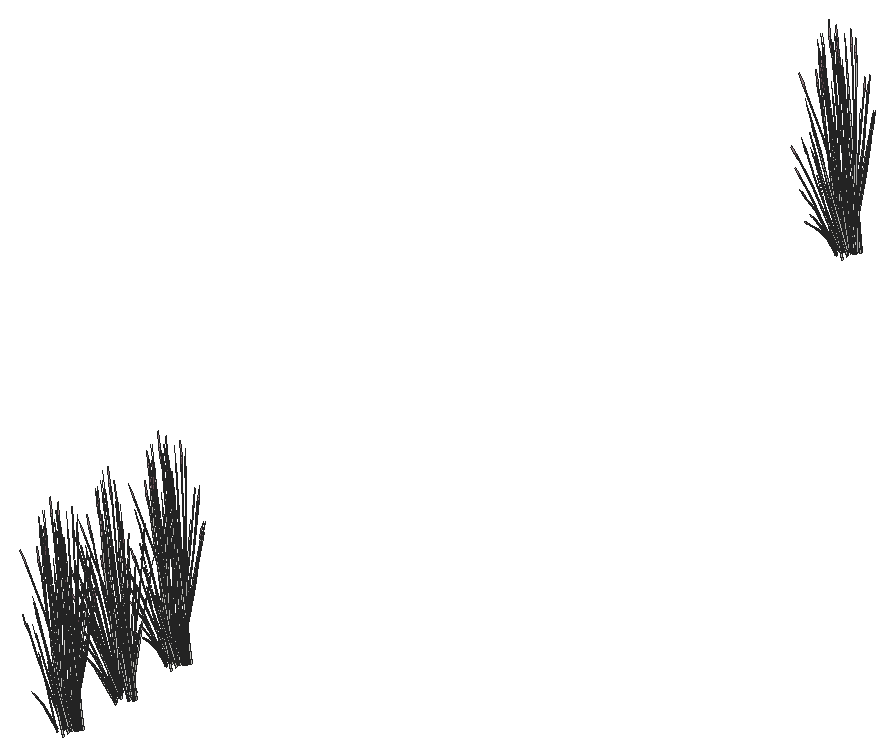
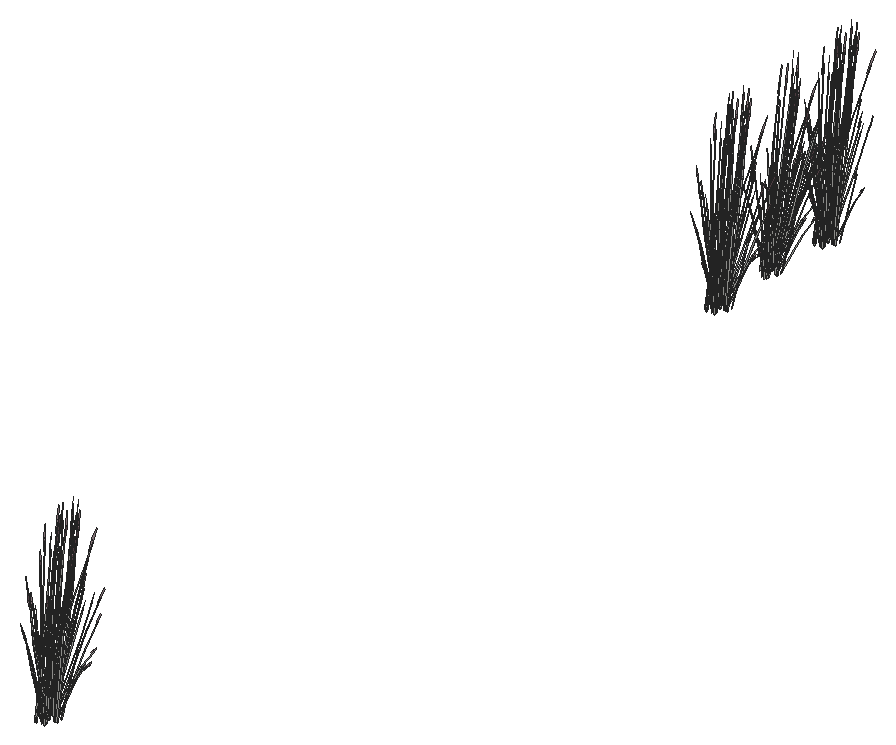
# SketchUp Ruby script. Lengths in inches.
U = 1.inch
M = Sketchup.active_model
def pt(a) = Geom::Point3d.new(a.map { |v| v * U })
def face(e, loops, mat)
  f = e.add_face(loops[0].map { |a| pt(a) })
  loops[1..].each { |l| e.add_face(l.map { |a| pt(a) }).erase! }
  f.material = f.back_material = mat if mat
  f
end
# faces: each face lists its corners as indices into pts; further lists are holes
def faces(e, pts, list, mat = nil) = list.each { |f| face(e, (f[0].is_a?(Array) ? f : [f]).map { |l| l.map { |i| pts[i] } }, mat) }
# xy, xz, yz: faces in a plane at the given z, y or x. An outline is a flat list of corners, or four numbers for a rectangle; further outlines are holes
def ring(l) = l.size == 4 ? [[l[0], l[1]], [l[2], l[1]], [l[2], l[3]], [l[0], l[3]]] : l.each_slice(2).to_a
def flat(e, list, mat, &to3) = list.each { |f| face(e, (f[0].is_a?(Array) ? f : [f]).map { |l| ring(l).map { |u, v| to3.(u, v) } }, mat) }
def xy(e, z, list, mat = nil) = flat(e, list, mat) { |x, y| [x, y, z] }
def xz(e, y, list, mat = nil) = flat(e, list, mat) { |x, z| [x, y, z] }
def yz(e, x, list, mat = nil) = flat(e, list, mat) { |y, z| [x, y, z] }
def lines(e, pts, list) = list.each { |a, b| e.add_line(pt(pts[a]), pt(pts[b])) }
# prism: a flat outline (further loops are holes) pulled along v
def prism(e, loops, v, mat = nil)
  f = face(e, loops, mat); d = Geom::Vector3d.new(v.map { |x| x * U })
  f.pushpull(f.normal.samedirection?(d) ? d.length : -d.length)
end
def box(e, o, s, mat = nil) = prism(e, [[o, [o[0] + s[0], o[1], o[2]], [o[0] + s[0], o[1] + s[1], o[2]], [o[0], o[1] + s[1], o[2]]]], [0, 0, s[2]], mat)
def at(x, y, z, deg = 0) = Geom::Transformation.translation(pt([x, y, z])) * Geom::Transformation.rotation(ORIGIN, Z_AXIS, deg.degrees)
def axes(o, x, y, z) = Geom::Transformation.new([*x, 0, *y, 0, *z, 0, *pt(o).to_a, 1])
def part(name) = M.definitions.add(name)
# library, detail: a bought-in or finely detailed component or shape, given as its bounding box
def library(name, o, s) = part(name).tap { |d| box(d.entities, o, s) }
def detail(e, o, s) = box(e.add_group.entities, o, s)
def put(e, d, t, mat = nil) = e.add_instance(d, t).tap { |i| i.material = mat if mat }
def group(e, t, mat = nil) = e.add_group.tap { |g| g.transformation = t; g.material = mat if mat }.entities
root = M.entities
M.materials.add("LightPink_Translucent").color = [144, 107, 117]
M.materials["LightPink_Translucent"].alpha = 0.75
c1 = part("blade")
p = [[2.15,0.21,22],[0,0.17,0],[0.09,0.45,0],[2.18,0.31,22],[2.29,0.31,22],[0.38,0.45,0],
  [2.48,0.24,33],[2.49,0.24,33],[2.48,0.22,33]]
faces(c1.entities,p,[[0,1,2,3],[4,5,2,3],[6,3,4,7],[8,0,3,6]])
c2 = part("seeds")
p = [[0.3,-0.1,1.38],[-0.01,-0.03,1.59],[-0.01,-0.03,0.03],[0.14,-0.07,-0.07],[0.29,-0.03,3],[0.15,0.01,3.11]]
faces(c2.entities,p,[[0,1,2,3],[1,0,4,5]],"LightPink_Translucent")
c3 = part("blade with seeds")
put(c3.entities,c1,at(0,0,0))
put(c3.entities,c2,axes([2.4,0.25,30.99],[1.5799,-0.05474,1.17369],[-0.12525,1.92788,0.29478],[-0.07173,-0.02425,1.56792]))
put(root,c3,axes([491.625,164.9375,4.29],[0.62747,-0.45094,0.53763],[0.54116,0.47889,0.4433],[-0.29439,-0.08318,1.11249]))
put(root,c3,axes([491.1,167.63,3.92],[-0.52161,-0.25698,0.0643],[0.30368,-0.36595,0.50621],[-0.16723,0.11831,0.77189]))
put(root,c3,axes([488.5,445.23,4.84],[0.67048,0.16311,-0.06488],[-0.20625,0.50201,-0.29416],[-0.10966,0.07622,0.97024]))
put(root,c3,axes([488.57,148.83,4.84],[0.67048,0.16311,-0.06488],[-0.20625,0.50201,-0.29416],[-0.10966,0.07622,0.97024]))
put(root,c3,axes([490,443.81,4.24],[0.66138,-0.08733,0.35414],[0.17464,0.49921,-0.4572],[-0.18953,0.13408,0.87481]))
put(root,c3,axes([488.64,189.9,4.84],[0.67048,0.16311,-0.06488],[-0.20625,0.50201,-0.29416],[-0.10966,0.07622,0.97024]))
put(root,c3,axes([490.08,147.41,4.24],[0.66138,-0.08733,0.35414],[0.17464,0.49921,-0.4572],[-0.18953,0.13408,0.87481]))
put(root,c3,axes([492.16,167.82,3.07],[0.14147,-0.21002,1.71376],[0.59349,0.43464,0.13857],[-0.26773,0.27089,0.73262]))
put(root,c3,axes([490.375,446.1875,1.78],[0.23977,-0.09639,1.43002],[0.59198,0.29065,-0.30754],[-0.1762,0.25149,0.61141]))
put(root,c3,axes([490.14,188.48,4.24],[0.66138,-0.08733,0.35414],[0.17464,0.49921,-0.4572],[-0.18953,0.13408,0.87481]))
put(root,c3,axes([490.04,440.69,1.32],[-0.21918,0.49894,-0.03893],[-0.6746,-0.15348,-0.17649],[-0.10242,-0.08161,0.58215]))
put(root,c3,axes([490.45,149.79,1.78],[0.23977,-0.09639,1.43002],[0.59198,0.29065,-0.30754],[-0.1762,0.25149,0.61141]))
put(root,c3,axes([490.52,190.86,1.78],[0.23977,-0.09639,1.43002],[0.59198,0.29065,-0.30754],[-0.1762,0.25149,0.61141]))
put(root,c3,axes([490.11,144.29,1.32],[-0.21918,0.49894,-0.03893],[-0.6746,-0.15348,-0.17649],[-0.10242,-0.08161,0.58215]))
put(root,c3,axes([491.59,166.36,4.24],[0.63144,0.17046,0.35414],[-0.18417,0.49731,-0.4572],[-0.25423,0.0456,0.87481]))
put(root,c3,axes([490.18,185.36,1.32],[-0.21918,0.49894,-0.03893],[-0.6746,-0.15348,-0.17649],[-0.10242,-0.08161,0.58215]))
put(root,c3,axes([491.79,439,3.9],[-0.01417,0.07324,1.77383],[-0.6991,0.2658,-0.16761],[-0.20573,-0.13587,0.31391]))
put(root,c3,axes([491.04,440.0625,1.78],[-0.04601,0.19989,1.43002],[-0.67263,0.16733,-0.30754],[-0.15723,-0.25836,0.61141]))
put(root,c3,axes([491.7,167.9,3.875],[0.19519,0.55794,-0.51099],[-0.73919,0.0976,-0.3958],[-0.21183,0.14986,0.97773]))
put(root,c3,axes([491.94,183.67,3.9],[-0.01417,0.07324,1.77383],[-0.6991,0.2658,-0.16761],[-0.20573,-0.13587,0.31391]))
put(root,c3,axes([491.26,440.58,3.07],[0.17368,0.19618,1.71376],[-0.80256,0.16516,0.13857],[-0.18139,-0.30799,0.73262]))
put(root,c3,axes([491.91,164.94,3.92],[0.03826,-0.46465,0.0643],[0.57772,0.01274,0.50621],[-0.2213,-0.04862,0.77189]))
put(root,c3,axes([490.55,168.9,3.91],[-0.01889,0.12092,1.74944],[0.53598,0.42065,-0.27667],[-0.14032,0.19892,0.14031]))
put(root,c3,axes([492.74,443.85,1.86],[-0.76714,0.40567,-0.29095],[-0.51013,-0.57321,-0.50002],[-0.18927,-0.05821,1.59708]))
put(root,c3,axes([491.19,184.73,1.78],[-0.04601,0.19989,1.43002],[-0.67263,0.16733,-0.30754],[-0.15723,-0.25836,0.61141]))
put(root,c3,axes([490.625,445.14,3.93],[-0.54105,-0.41691,0.48003],[0.57458,-0.35956,0.3958],[-0.0998,0.1956,0.9933]))
put(root,c3,axes([493.54,167.5,1.25],[-0.79037,-0.10018,-0.62353],[0.16679,-0.61794,-0.16365],[-0.23587,-0.07488,1.37633]))
put(root,c3,axes([493.6875,164.13,4.62],[-0.50709,0.58578,-0.13619],[-0.73436,-0.33748,-0.75594],[-0.25527,-0.1655,1.14864]))
put(root,c3,axes([492.82,147.46,1.86],[-0.76714,0.40567,-0.29095],[-0.51013,-0.57321,-0.50002],[-0.18927,-0.05821,1.59708]))
put(root,c3,axes([491.41,185.25,3.07],[0.17368,0.19618,1.71376],[-0.80256,0.16516,0.13857],[-0.18139,-0.30799,0.73262]))
put(root,c3,axes([490.7,148.74,3.93],[-0.54105,-0.41691,0.48003],[0.57458,-0.35956,0.3958],[-0.0998,0.1956,0.9933]))
put(root,c3,axes([491.54,440.48,3.72],[-0.11735,-0.49217,-0.35414],[0.67083,-0.12996,0.4572],[-0.18018,-0.14104,0.87481]))
put(root,c3,axes([492.89,188.52,1.86],[-0.76714,0.40567,-0.29095],[-0.51013,-0.57321,-0.50002],[-0.18927,-0.05821,1.59708]))
put(root,c3,axes([492.3,165.28,4.24],[0.43232,0.38257,0.35414],[-0.49364,0.36215,-0.4572],[-0.25081,-0.0551,0.87481]))
put(root,c3,axes([490.77,189.81,3.93],[-0.54105,-0.41691,0.48003],[0.57458,-0.35956,0.3958],[-0.0998,0.1956,0.9933]))
put(root,c3,axes([489.67,442.97,1.57],[-0.95008,0,0],[0,-0.68292,-0.51607],[0,-0.15554,1.63711]))
put(root,c3,axes([491.01,444.7,1.22],[-0.17848,-0.53243,-0.30978],[0.70886,-0.15119,0.30978],[-0.1429,-0.0614,1.38974]))
put(root,c3,axes([491.62,144.08,3.72],[-0.11735,-0.49217,-0.35414],[0.67083,-0.12996,0.4572],[-0.18018,-0.14104,0.87481]))
put(root,c3,axes([490.43,445.1,3.92],[-0.62439,-0.02847,0.0643],[0.01712,-0.42991,0.50621],[-0.06534,0.16468,0.77189]))
put(root,c3,axes([493.47,164.61,4.17],[-0.64788,-0.29534,-0.71045],[0.46044,-0.51755,0.08574],[-0.23473,-0.17635,1.00501]))
put(root,c3,axes([489.75,146.57,1.57],[-0.95008,0,0],[0,-0.68292,-0.51607],[0,-0.15554,1.63711]))
put(root,c3,axes([491.09,148.31,1.22],[-0.17848,-0.53243,-0.30978],[0.70886,-0.15119,0.30978],[-0.1429,-0.0614,1.38974]))
put(root,c3,axes([491.69,185.15,3.72],[-0.11735,-0.49217,-0.35414],[0.67083,-0.12996,0.4572],[-0.18018,-0.14104,0.87481]))
put(root,c3,axes([493.16,164.62,3.875],[-0.74975,0.14525,-0.51099],[-0.13115,-0.55007,-0.3958],[-0.20138,-0.15763,0.97773]))
put(root,c3,axes([490.5,148.7,3.92],[-0.62439,-0.02847,0.0643],[0.01712,-0.42991,0.50621],[-0.06534,0.16468,0.77189]))
put(root,c3,axes([490.62,445.26,3.72],[-0.5141,0.32171,-0.35414],[-0.48666,-0.36734,0.4572],[-0.07405,0.18664,0.87481]))
put(root,c3,axes([489.82,187.64,1.57],[-0.95008,0,0],[0,-0.68292,-0.51607],[0,-0.15554,1.63711]))
put(root,c3,axes([491.15,189.375,1.22],[-0.17848,-0.53243,-0.30978],[0.70886,-0.15119,0.30978],[-0.1429,-0.0614,1.38974]))
put(root,c3,axes([490.57,189.77,3.92],[-0.62439,-0.02847,0.0643],[0.01712,-0.42991,0.50621],[-0.06534,0.16468,0.77189]))
put(root,c3,axes([490.7,148.86,3.72],[-0.5141,0.32171,-0.35414],[-0.48666,-0.36734,0.4572],[-0.07405,0.18664,0.87481]))
put(root,c3,axes([490.77,189.93,3.72],[-0.5141,0.32171,-0.35414],[-0.48666,-0.36734,0.4572],[-0.07405,0.18664,0.87481]))
put(root,c3,axes([492.51,168.67,1.21],[-0.7111,-0.30552,-0.49651],[0.42504,-0.54784,0],[-0.16196,-0.06958,1.57504]))
put(root,c3,axes([493.25,444.3,1.25],[-0.51177,0.45928,-0.62353],[-0.63575,-0.41646,-0.16365],[-0.20507,0.11457,1.37633]))
put(root,c3,axes([492.19,164.12,0.6875],[-0.0736,0.08049,1.76342],[-0.74378,0.17355,-0.26939],[-0.17968,-0.15788,0.30037]))
put(root,c3,axes([491.35,167.5,4.23],[0.70283,0.33692,-0.1216],[-0.40491,0.48793,-0.67495],[-0.19857,0.16961,1.02557]))
put(root,c3,axes([491.94,440.88,4.24],[0.11735,0.49217,0.35414],[-0.67083,0.12996,-0.4572],[-0.18018,-0.14104,0.87481]))
put(root,c3,axes([493.33,147.9,1.25],[-0.51177,0.45928,-0.62353],[-0.63575,-0.41646,-0.16365],[-0.20507,0.11457,1.37633]))
put(root,c3,axes([488.79,446.41,3.9],[0.0862,-0.03689,1.77383],[0.71245,0.24539,-0.16761],[-0.01674,0.20431,0.31391]))
put(root,c3,axes([492.02,144.48,4.24],[0.11735,0.49217,0.35414],[-0.67083,0.12996,-0.4572],[-0.18018,-0.14104,0.87481]))
put(root,c3,axes([490.41,442.79,1.52],[-0.70674,0.51372,0.30756],[-0.70717,-0.50832,-0.36492],[-0.02468,-0.14589,1.64885]))
put(root,c3,axes([492.94,169.04,1.57],[-0.47504,0.61229,0],[-0.79476,-0.34146,-0.51607],[-0.18101,-0.07777,1.63711]))
put(root,c3,axes([493.4,188.97,1.25],[-0.51177,0.45928,-0.62353],[-0.63575,-0.41646,-0.16365],[-0.20507,0.11457,1.37633]))
put(root,c3,axes([488.87,150.01,3.9],[0.0862,-0.03689,1.77383],[0.71245,0.24539,-0.16761],[-0.01674,0.20431,0.31391]))
put(root,c3,axes([492.09,185.55,4.24],[0.11735,0.49217,0.35414],[-0.67083,0.12996,-0.4572],[-0.18018,-0.14104,0.87481]))
put(root,c3,axes([490.49,146.39,1.52],[-0.70674,0.51372,0.30756],[-0.70717,-0.50832,-0.36492],[-0.02468,-0.14589,1.64885]))
put(root,c3,axes([488.9375,191.08,3.9],[0.0862,-0.03689,1.77383],[0.71245,0.24539,-0.16761],[-0.01674,0.20431,0.31391]))
put(root,c3,axes([493.32,444.21,2.52],[0.65659,0.2464,1.51261],[-0.64324,0.53082,0.59816],[-0.28812,-0.31461,1.26806]))
put(root,c3,axes([490.56,187.46,1.52],[-0.70674,0.51372,0.30756],[-0.70717,-0.50832,-0.36492],[-0.02468,-0.14589,1.64885]))
put(root,c3,axes([493.4,147.81,2.52],[0.65659,0.2464,1.51261],[-0.64324,0.53082,0.59816],[-0.28812,-0.31461,1.26806]))
put(root,c3,axes([490.8125,439.74,1.96],[0.39634,0.21267,1.1486],[-0.57721,0.12784,0.84392],[-0.1235,-0.16344,0.25299]))
put(root,c3,axes([493.61,444.04,1.66],[-0.74193,-0.49181,-0.25192],[0.6243,-0.55226,0.5513],[-0.19979,0.05753,1.68216]))
put(root,c3,axes([493.47,188.88,2.52],[0.65659,0.2464,1.51261],[-0.64324,0.53082,0.59816],[-0.28812,-0.31461,1.26806]))
put(root,c3,axes([492.26,443.57,1.4],[-0.45644,-0.51287,-0.44739],[0.69137,-0.36116,0.21531],[-0.14771,-0.06346,1.43643]))
put(root,c3,axes([490.89,143.34,1.96],[0.39634,0.21267,1.1486],[-0.57721,0.12784,0.84392],[-0.1235,-0.16344,0.25299]))
put(root,c3,axes([493.68,147.64,1.66],[-0.74193,-0.49181,-0.25192],[0.6243,-0.55226,0.5513],[-0.19979,0.05753,1.68216]))
put(root,c3,axes([490.19,168.97,4.84],[0.67048,0.16311,-0.06488],[-0.20625,0.50201,-0.29416],[-0.10966,0.07622,0.97024]))
put(root,c3,axes([492.33,147.17,1.4],[-0.45644,-0.51287,-0.44739],[0.69137,-0.36116,0.21531],[-0.14771,-0.06346,1.43643]))
put(root,c3,axes([490.97,444.92,4.53],[-0.01977,0.56521,-0.7886],[-0.83252,-0.03796,0.09517],[-0.08786,0.23945,1.11556]))
put(root,c3,axes([490.96,184.41,1.96],[0.39634,0.21267,1.1486],[-0.57721,0.12784,0.84392],[-0.1235,-0.16344,0.25299]))
put(root,c3,axes([493.75,188.71,1.66],[-0.74193,-0.49181,-0.25192],[0.6243,-0.55226,0.5513],[-0.19979,0.05753,1.68216]))
put(root,c3,axes([492.4,188.24,1.4],[-0.45644,-0.51287,-0.44739],[0.69137,-0.36116,0.21531],[-0.14771,-0.06346,1.43643]))
put(root,c3,axes([491.04,148.52,4.53],[-0.01977,0.56521,-0.7886],[-0.83252,-0.03796,0.09517],[-0.08786,0.23945,1.11556]))
put(root,c3,axes([491.7,167.55,4.24],[0.66138,-0.08733,0.35414],[0.17464,0.49921,-0.4572],[-0.18953,0.13408,0.87481]))
put(root,c3,axes([490.95,446.51,1.96],[-0.01966,-0.36332,1.1486],[0.49135,0.25914,0.84392],[-0.09663,0.17317,0.25299]))
put(root,c3,axes([491.64,440.3,4.29],[0.84639,-0.15705,0.53763],[0.14689,0.61608,0.4433],[-0.19906,-0.18157,1.11249]))
put(root,c3,axes([491.11,189.59,4.53],[-0.01977,0.56521,-0.7886],[-0.83252,-0.03796,0.09517],[-0.08786,0.23945,1.11556]))
put(root,c3,axes([493.23,443.94,1.4],[-0.82508,0.03772,-0.44739],[-0.07462,-0.62614,0.21531],[-0.14771,0.06346,1.43643]))
put(root,c3,axes([491.03,150.11,1.96],[-0.01966,-0.36332,1.1486],[0.49135,0.25914,0.84392],[-0.09663,0.17317,0.25299]))
put(root,c3,axes([492.07,169.93,1.78],[0.23977,-0.09639,1.43002],[0.59198,0.29065,-0.30754],[-0.1762,0.25149,0.61141]))
put(root,c3,axes([491.1,191.18,1.96],[-0.01966,-0.36332,1.1486],[0.49135,0.25914,0.84392],[-0.09663,0.17317,0.25299]))
put(root,c3,axes([491.73,164.43,1.32],[-0.21918,0.49894,-0.03893],[-0.6746,-0.15348,-0.17649],[-0.10242,-0.08161,0.58215]))
put(root,c3,axes([493.31,147.54,1.4],[-0.82508,0.03772,-0.44739],[-0.07462,-0.62614,0.21531],[-0.14771,0.06346,1.43643]))
put(root,c3,axes([491.79,184.97,4.29],[0.84639,-0.15705,0.53763],[0.14689,0.61608,0.4433],[-0.19906,-0.18157,1.11249]))
put(root,c3,axes([493.375,188.61,1.4],[-0.82508,0.03772,-0.44739],[-0.07462,-0.62614,0.21531],[-0.14771,0.06346,1.43643]))
put(root,c3,axes([491.83,440.43,3.92],[0.34533,-0.38816,0.0643],[0.49176,0.22599,0.50621],[-0.15898,-0.12445,0.77189]))
put(root,c3,axes([493.49,162.74,3.9],[-0.01417,0.07324,1.77383],[-0.6991,0.2658,-0.16761],[-0.20573,-0.13587,0.31391]))
put(root,c3,axes([491.91,144.03,3.92],[0.34533,-0.38816,0.0643],[0.49176,0.22599,0.50621],[-0.15898,-0.12445,0.77189]))
put(root,c3,axes([491.65,444.98,1.67],[0.7111,0.30552,0.49651],[-0.42504,0.54784,0],[-0.16196,-0.06958,1.57504]))
put(root,c3,axes([490.6875,445.72,2.56],[0.01669,-0.31544,1.54345],[0.75083,0.16661,0.21329],[-0.06506,0.33618,0.72882]))
put(root,c3,axes([492.74,163.8,1.78],[-0.04601,0.19989,1.43002],[-0.67263,0.16733,-0.30754],[-0.15723,-0.25836,0.61141]))
put(root,c3,axes([491.98,185.1,3.92],[0.34533,-0.38816,0.0643],[0.49176,0.22599,0.50621],[-0.15898,-0.12445,0.77189]))
put(root,c3,axes([491.73,148.58,1.67],[0.7111,0.30552,0.49651],[-0.42504,0.54784,0],[-0.16196,-0.06958,1.57504]))
put(root,c3,axes([492.96,164.32,3.07],[0.17368,0.19618,1.71376],[-0.80256,0.16516,0.13857],[-0.18139,-0.30799,0.73262]))
put(root,c3,axes([490.76,149.32,2.56],[0.01669,-0.31544,1.54345],[0.75083,0.16661,0.21329],[-0.06506,0.33618,0.72882]))
put(root,c3,axes([492.32,443.86,1.63],[0.20138,-0.72405,-0.23429],[0.95485,0.12621,0.51271],[-0.16685,-0.09999,1.5644]))
put(root,c3,axes([494.44,167.59,1.86],[-0.76714,0.40567,-0.29095],[-0.51013,-0.57321,-0.50002],[-0.18927,-0.05821,1.59708]))
put(root,c3,axes([491.8,189.65,1.67],[0.7111,0.30552,0.49651],[-0.42504,0.54784,0],[-0.16196,-0.06958,1.57504]))
put(root,c3,axes([490.83,190.39,2.56],[0.01669,-0.31544,1.54345],[0.75083,0.16661,0.21329],[-0.06506,0.33618,0.72882]))
put(root,c3,axes([492.32,168.875,3.93],[-0.54105,-0.41691,0.48003],[0.57458,-0.35956,0.3958],[-0.0998,0.1956,0.9933]))
put(root,c3,axes([492.4,147.46,1.63],[0.20138,-0.72405,-0.23429],[0.95485,0.12621,0.51271],[-0.16685,-0.09999,1.5644]))
put(root,c3,axes([492.47,188.53,1.63],[0.20138,-0.72405,-0.23429],[0.95485,0.12621,0.51271],[-0.16685,-0.09999,1.5644]))
put(root,c3,axes([493.24,164.22,3.72],[-0.11735,-0.49217,-0.35414],[0.67083,-0.12996,0.4572],[-0.18018,-0.14104,0.87481]))
put(root,c3,axes([492.67,444.03,1.81],[-0.14658,0.54532,0.1448],[-0.71613,-0.09466,-0.41347],[-0.13033,-0.05599,1.26744]))
put(root,c3,axes([491.37,166.71,1.57],[-0.95008,0,0],[0,-0.68292,-0.51607],[0,-0.15554,1.63711]))
put(root,c3,axes([492.71,168.44,1.22],[-0.17848,-0.53243,-0.30978],[0.70886,-0.15119,0.30978],[-0.1429,-0.0614,1.38974]))
put(root,c3,axes([492.59,439.28,3.91],[-0.11621,-0.08567,1.74944],[-0.77555,0.05431,-0.27667],[-0.12378,-0.20491,0.14031]))
put(root,c3,axes([492.75,147.63,1.81],[-0.14658,0.54532,0.1448],[-0.71613,-0.09466,-0.41347],[-0.13033,-0.05599,1.26744]))
put(root,c3,axes([492.12,168.84,3.92],[-0.62439,-0.02847,0.0643],[0.01712,-0.42991,0.50621],[-0.06534,0.16468,0.77189]))
put(root,c3,axes([494.1,445.55,1.21],[-0.7111,0.30552,-0.49651],[-0.42504,-0.54784,0],[-0.16196,0.06958,1.57504]))
put(root,c3,axes([489.89,442.51,1.21],[0,-0.61104,-0.49651],[0.85008,0,0],[0,-0.13917,1.57504]))
put(root,c3,axes([490.25,443.07,1.67],[0,0.61104,0.49651],[-0.85008,0,0],[0,-0.13917,1.57504]))
put(root,c3,axes([494.14,445.39,1.39],[-0.46912,-0.61443,-0.05142],[0.79476,-0.34146,0.51607],[-0.19584,0.0585,1.6363]))
put(root,c3,axes([492.82,188.7,1.81],[-0.14658,0.54532,0.1448],[-0.71613,-0.09466,-0.41347],[-0.13033,-0.05599,1.26744]))
put(root,c3,axes([494.17,149.15,1.21],[-0.7111,0.30552,-0.49651],[-0.42504,-0.54784,0],[-0.16196,0.06958,1.57504]))
put(root,c3,axes([492.32,169,3.72],[-0.5141,0.32171,-0.35414],[-0.48666,-0.36734,0.4572],[-0.07405,0.18664,0.87481]))
put(root,c3,axes([489.96,146.11,1.21],[0,-0.61104,-0.49651],[0.85008,0,0],[0,-0.13917,1.57504]))
put(root,c3,axes([490.33,146.67,1.67],[0,0.61104,0.49651],[-0.85008,0,0],[0,-0.13917,1.57504]))
put(root,c3,axes([494.22,148.99,1.39],[-0.46912,-0.61443,-0.05142],[0.79476,-0.34146,0.51607],[-0.19584,0.0585,1.6363]))
put(root,c3,axes([492.74,183.95,3.91],[-0.11621,-0.08567,1.74944],[-0.77555,0.05431,-0.27667],[-0.12378,-0.20491,0.14031]))
put(root,c3,axes([494.24,190.22,1.21],[-0.7111,0.30552,-0.49651],[-0.42504,-0.54784,0],[-0.16196,0.06958,1.57504]))
put(root,c3,axes([490.03,187.18,1.21],[0,-0.61104,-0.49651],[0.85008,0,0],[0,-0.13917,1.57504]))
put(root,c3,axes([490.4,187.74,1.67],[0,0.61104,0.49651],[-0.85008,0,0],[0,-0.13917,1.57504]))
put(root,c3,axes([494.29,190.06,1.39],[-0.46912,-0.61443,-0.05142],[0.79476,-0.34146,0.51607],[-0.19584,0.0585,1.6363]))
put(root,c3,axes([491.13,445.11,4.2],[0.54391,0.41056,-0.5672],[-0.57458,0.35956,-0.43934],[-0.08276,0.2086,1.08528]))
put(root,c3,axes([493.93,445.31,1.22],[-0.70886,-0.15119,-0.30978],[0.17848,-0.53243,0.30978],[-0.1429,0.0614,1.38974]))
put(root,c3,axes([494.95,168.04,1.25],[-0.51177,0.45928,-0.62353],[-0.63575,-0.41646,-0.16365],[-0.20507,0.11457,1.37633]))
put(root,c3,axes([491.21,148.71,4.2],[0.54391,0.41056,-0.5672],[-0.57458,0.35956,-0.43934],[-0.08276,0.2086,1.08528]))
put(root,c3,axes([490.89,444.8,4.24],[0.5141,-0.32171,0.35414],[0.48666,0.36734,-0.4572],[-0.07405,0.18664,0.87481]))
put(root,c3,axes([493.64,164.62,4.24],[0.11735,0.49217,0.35414],[-0.67083,0.12996,-0.4572],[-0.18018,-0.14104,0.87481]))
put(root,c3,axes([494.01,148.91,1.22],[-0.70886,-0.15119,-0.30978],[0.17848,-0.53243,0.30978],[-0.1429,0.0614,1.38974]))
put(root,c3,axes([491.28,189.78,4.2],[0.54391,0.41056,-0.5672],[-0.57458,0.35956,-0.43934],[-0.08276,0.2086,1.08528]))
put(root,c3,axes([490.49,170.14,3.9],[0.0862,-0.03689,1.77383],[0.71245,0.24539,-0.16761],[-0.01674,0.20431,0.31391]))
put(root,c3,axes([490.97,148.41,4.24],[0.5141,-0.32171,0.35414],[0.48666,0.36734,-0.4572],[-0.07405,0.18664,0.87481]))
put(root,c3,axes([492.11,443.21,1.86],[-0.85568,-0.29155,-0.29095],[0.41201,-0.61537,-0.50002],[-0.02689,-0.15109,1.59708]))
put(root,c3,axes([494.34,443.03,2.03],[-0.02076,-0.57531,1.41272],[0.93937,0.14913,0.59816],[-0.22217,0.31481,1.3335]))
put(root,c3,axes([492.11,166.53,1.52],[-0.70674,0.51372,0.30756],[-0.70717,-0.50832,-0.36492],[-0.02468,-0.14589,1.64885]))
put(root,c3,axes([494.08,189.98,1.22],[-0.70886,-0.15119,-0.30978],[0.17848,-0.53243,0.30978],[-0.1429,0.0614,1.38974]))
put(root,c3,axes([491.04,189.47,4.24],[0.5141,-0.32171,0.35414],[0.48666,0.36734,-0.4572],[-0.07405,0.18664,0.87481]))
put(root,c3,axes([492.19,146.8125,1.86],[-0.85568,-0.29155,-0.29095],[0.41201,-0.61537,-0.50002],[-0.02689,-0.15109,1.59708]))
put(root,c3,axes([494.41,146.63,2.03],[-0.02076,-0.57531,1.41272],[0.93937,0.14913,0.59816],[-0.22217,0.31481,1.3335]))
put(root,c3,axes([495.02,167.95,2.52],[0.65659,0.2464,1.51261],[-0.64324,0.53082,0.59816],[-0.28812,-0.31461,1.26806]))
put(root,c3,axes([492.25,187.88,1.86],[-0.85568,-0.29155,-0.29095],[0.41201,-0.61537,-0.50002],[-0.02689,-0.15109,1.59708]))
put(root,c3,axes([494.48,187.7,2.03],[-0.02076,-0.57531,1.41272],[0.93937,0.14913,0.59816],[-0.22217,0.31481,1.3335]))
put(root,c3,axes([490.5625,444.89,4.59],[0.83505,0.03027,-0.13498],[-0.02282,0.57322,-0.74919],[-0.05801,0.22077,1.13838]))
put(root,c3,axes([492.51,163.48,1.96],[0.39634,0.21267,1.1486],[-0.57721,0.12784,0.84392],[-0.1235,-0.16344,0.25299]))
put(root,c3,axes([495.3,167.78,1.66],[-0.74193,-0.49181,-0.25192],[0.6243,-0.55226,0.5513],[-0.19979,0.05753,1.68216]))
put(root,c3,axes([493.95,167.31,1.4],[-0.45644,-0.51287,-0.44739],[0.69137,-0.36116,0.21531],[-0.14771,-0.06346,1.43643]))
put(root,c3,axes([490.54,445.73,2.02],[0.69024,-0.1082,0.06507],[0.15868,0.43593,-0.86304],[-0.04376,0.22067,0.7736]))
put(root,c3,axes([490.64,148.49,4.59],[0.83505,0.03027,-0.13498],[-0.02282,0.57322,-0.74919],[-0.05801,0.22077,1.13838]))
put(root,c3,axes([493.81,443.77,1.86],[0.08854,0.69723,-0.29095],[-0.92215,0.04216,-0.50002],[-0.16238,0.09287,1.59708]))
put(root,c3,axes([491.73,442.59,1.29],[-0.31203,-0.62659,-0.69835],[0.89884,-0.22566,-0.18329],[-0.03449,-0.21218,1.54149]))
put(root,c3,axes([493.77,440.6,4.23],[-0.74352,0.28449,-0.1216],[-0.36538,-0.50492,-0.67495],[-0.0981,-0.21277,1.02557]))
put(root,c3,axes([490.62,149.33,2.02],[0.69024,-0.1082,0.06507],[0.15868,0.43593,-0.86304],[-0.04376,0.22067,0.7736]))
put(root,c3,axes([490.71,189.5625,4.59],[0.83505,0.03027,-0.13498],[-0.02282,0.57322,-0.74919],[-0.05801,0.22077,1.13838]))
put(root,c3,axes([493.13,440.63,3.875],[-0.7469,-0.15318,-0.51099],[0.25601,-0.52518,-0.3958],[-0.06849,-0.21144,0.97773]))
put(root,c3,axes([492.66,168.66,4.53],[-0.01977,0.56521,-0.7886],[-0.83252,-0.03796,0.09517],[-0.08786,0.23945,1.11556]))
put(root,c3,axes([493.89,147.37,1.86],[0.08854,0.69723,-0.29095],[-0.92215,0.04216,-0.50002],[-0.16238,0.09287,1.59708]))
put(root,c3,axes([491.8,146.19,1.29],[-0.31203,-0.62659,-0.69835],[0.89884,-0.22566,-0.18329],[-0.03449,-0.21218,1.54149]))
put(root,c3,axes([493.85,144.2,4.23],[-0.74352,0.28449,-0.1216],[-0.36538,-0.50492,-0.67495],[-0.0981,-0.21277,1.02557]))
put(root,c3,axes([490.69,190.4,2.02],[0.69024,-0.1082,0.06507],[0.15868,0.43593,-0.86304],[-0.04376,0.22067,0.7736]))
put(root,c3,axes([493.95,188.44,1.86],[0.08854,0.69723,-0.29095],[-0.92215,0.04216,-0.50002],[-0.16238,0.09287,1.59708]))
put(root,c3,axes([492.65,170.25,1.96],[-0.01966,-0.36332,1.1486],[0.49135,0.25914,0.84392],[-0.09663,0.17317,0.25299]))
put(root,c3,axes([491.87,187.26,1.29],[-0.31203,-0.62659,-0.69835],[0.89884,-0.22566,-0.18329],[-0.03449,-0.21218,1.54149]))
put(root,c3,axes([493.34,164.04,4.29],[0.84639,-0.15705,0.53763],[0.14689,0.61608,0.4433],[-0.19906,-0.18157,1.11249]))
put(root,c3,axes([491.75,444.52,3.07],[-0.0186,-0.23452,1.71376],[0.80601,0.15558,0.13857],[-0.04985,0.33422,0.73262]))
put(root,c3,axes([493.92,185.27,4.23],[-0.74352,0.28449,-0.1216],[-0.36538,-0.50492,-0.67495],[-0.0981,-0.21277,1.02557]))
put(root,c3,axes([493.28,185.3,3.875],[-0.7469,-0.15318,-0.51099],[0.25601,-0.52518,-0.3958],[-0.06849,-0.21144,0.97773]))
put(root,c3,axes([494.93,167.67,1.4],[-0.82508,0.03772,-0.44739],[-0.07462,-0.62614,0.21531],[-0.14771,0.06346,1.43643]))
put(root,c3,axes([491.83,148.12,3.07],[-0.0186,-0.23452,1.71376],[0.80601,0.15558,0.13857],[-0.04985,0.33422,0.73262]))
put(root,c3,axes([490.25,442.52,1.22],[0.53038,-0.38124,-0.30978],[0.53038,0.38124,0.30978],[0,-0.1228,1.38974]))
put(root,c3,axes([491.9,189.19,3.07],[-0.0186,-0.23452,1.71376],[0.80601,0.15558,0.13857],[-0.04985,0.33422,0.73262]))
put(root,c3,axes([492.65,440.05,1.32],[-0.52505,0.35054,-0.03893],[-0.48109,-0.38392,-0.17649],[-0.03387,-0.10878,0.58215]))
put(root,c3,axes([490.33,146.12,1.22],[0.53038,-0.38124,-0.30978],[0.53038,0.38124,0.30978],[0,-0.1228,1.38974]))
put(root,c3,axes([492.43,443.51,1.55],[0.96033,0.12874,0.45755],[-0.19544,0.7271,0.17955],[-0.14034,-0.07021,1.58856]))
put(root,c3,axes([493.53,164.17,3.92],[0.34533,-0.38816,0.0643],[0.49176,0.22599,0.50621],[-0.15898,-0.12445,0.77189]))
put(root,c3,axes([492.72,143.66,1.32],[-0.52505,0.35054,-0.03893],[-0.48109,-0.38392,-0.17649],[-0.03387,-0.10878,0.58215]))
put(root,c3,axes([490.4,187.19,1.22],[0.53038,-0.38124,-0.30978],[0.53038,0.38124,0.30978],[0,-0.1228,1.38974]))
put(root,c3,axes([492.51,147.11,1.55],[0.96033,0.12874,0.45755],[-0.19544,0.7271,0.17955],[-0.14034,-0.07021,1.58856]))
put(root,c3,axes([492.79,184.72,1.32],[-0.52505,0.35054,-0.03893],[-0.48109,-0.38392,-0.17649],[-0.03387,-0.10878,0.58215]))
put(root,c3,axes([493.35,168.72,1.67],[0.7111,0.30552,0.49651],[-0.42504,0.54784,0],[-0.16196,-0.06958,1.57504]))
put(root,c3,axes([492.38,169.46,2.56],[0.01669,-0.31544,1.54345],[0.75083,0.16661,0.21329],[-0.06506,0.33618,0.72882]))
put(root,c3,axes([492.58,188.18,1.55],[0.96033,0.12874,0.45755],[-0.19544,0.7271,0.17955],[-0.14034,-0.07021,1.58856]))
